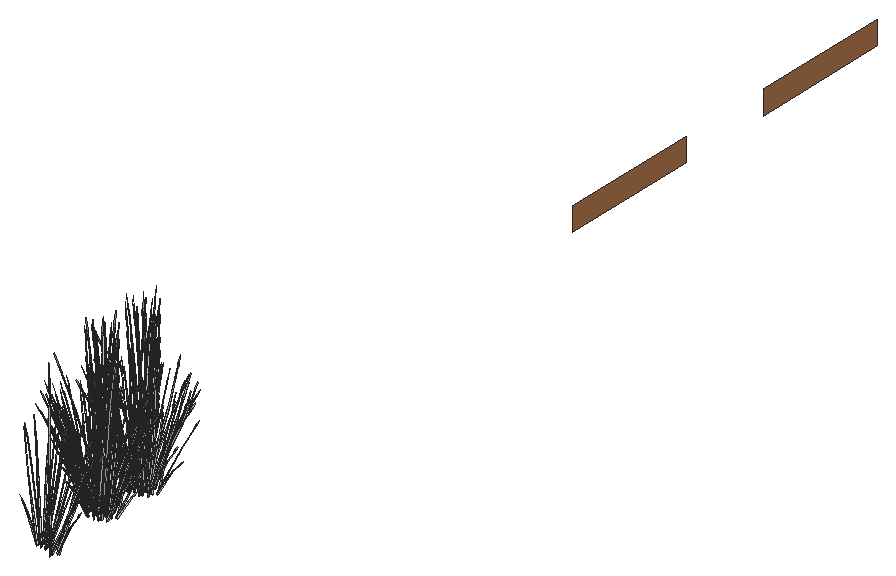
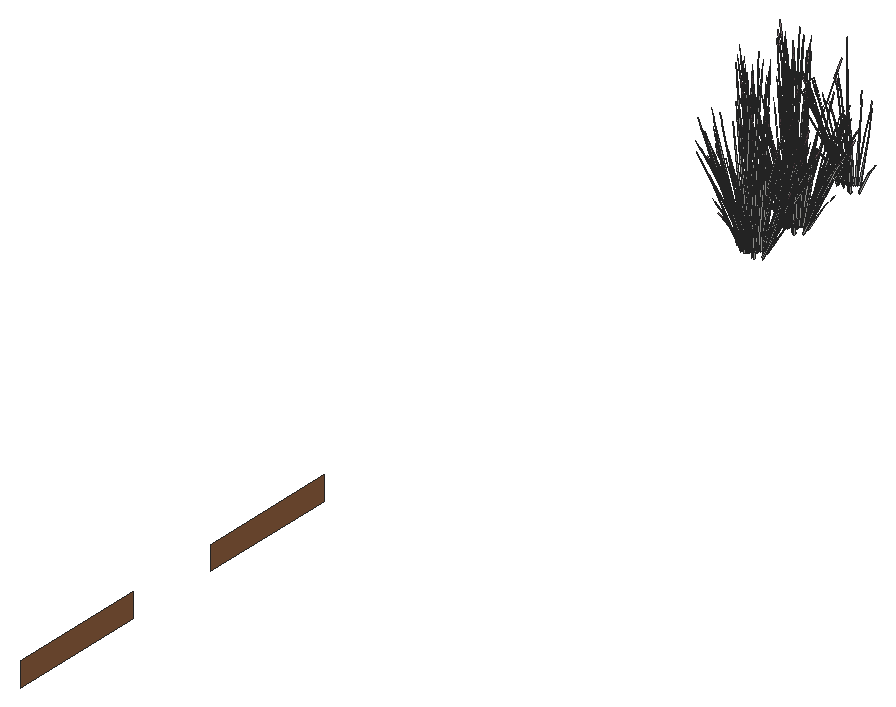
# SketchUp Ruby script. Lengths in inches.
U = 1.inch
M = Sketchup.active_model
def pt(a) = Geom::Point3d.new(a.map { |v| v * U })
def face(e, loops, mat)
  f = e.add_face(loops[0].map { |a| pt(a) })
  loops[1..].each { |l| e.add_face(l.map { |a| pt(a) }).erase! }
  f.material = f.back_material = mat if mat
  f
end
# faces: each face lists its corners as indices into pts; further lists are holes
def faces(e, pts, list, mat = nil) = list.each { |f| face(e, (f[0].is_a?(Array) ? f : [f]).map { |l| l.map { |i| pts[i] } }, mat) }
# xy, xz, yz: faces in a plane at the given z, y or x. An outline is a flat list of corners, or four numbers for a rectangle; further outlines are holes
def ring(l) = l.size == 4 ? [[l[0], l[1]], [l[2], l[1]], [l[2], l[3]], [l[0], l[3]]] : l.each_slice(2).to_a
def flat(e, list, mat, &to3) = list.each { |f| face(e, (f[0].is_a?(Array) ? f : [f]).map { |l| ring(l).map { |u, v| to3.(u, v) } }, mat) }
def xy(e, z, list, mat = nil) = flat(e, list, mat) { |x, y| [x, y, z] }
def xz(e, y, list, mat = nil) = flat(e, list, mat) { |x, z| [x, y, z] }
def yz(e, x, list, mat = nil) = flat(e, list, mat) { |y, z| [x, y, z] }
def lines(e, pts, list) = list.each { |a, b| e.add_line(pt(pts[a]), pt(pts[b])) }
# prism: a flat outline (further loops are holes) pulled along v
def prism(e, loops, v, mat = nil)
  f = face(e, loops, mat); d = Geom::Vector3d.new(v.map { |x| x * U })
  f.pushpull(f.normal.samedirection?(d) ? d.length : -d.length)
end
def box(e, o, s, mat = nil) = prism(e, [[o, [o[0] + s[0], o[1], o[2]], [o[0] + s[0], o[1] + s[1], o[2]], [o[0], o[1] + s[1], o[2]]]], [0, 0, s[2]], mat)
def at(x, y, z, deg = 0) = Geom::Transformation.translation(pt([x, y, z])) * Geom::Transformation.rotation(ORIGIN, Z_AXIS, deg.degrees)
def axes(o, x, y, z) = Geom::Transformation.new([*x, 0, *y, 0, *z, 0, *pt(o).to_a, 1])
def part(name) = M.definitions.add(name)
# library, detail: a bought-in or finely detailed component or shape, given as its bounding box
def library(name, o, s) = part(name).tap { |d| box(d.entities, o, s) }
def detail(e, o, s) = box(e.add_group.entities, o, s)
def put(e, d, t, mat = nil) = e.add_instance(d, t).tap { |i| i.material = mat if mat }
def group(e, t, mat = nil) = e.add_group.tap { |g| g.transformation = t; g.material = mat if mat }.entities
root = M.entities
M.materials.add("LightPink_Translucent").color = [144, 107, 117]
M.materials["LightPink_Translucent"].alpha = 0.75
M.materials.add("Wood_Veneer_15_1K").color = [163, 109, 71]
c1 = part("blade")
p = [[2.15,0.21,22],[0,0.17,0],[0.09,0.45,0],[2.18,0.31,22],[2.29,0.31,22],[0.38,0.45,0],
  [2.48,0.24,33],[2.49,0.24,33],[2.48,0.22,33]]
faces(c1.entities,p,[[0,1,2,3],[4,5,2,3],[6,3,4,7],[8,0,3,6]])
c2 = part("seeds")
p = [[0.3,-0.1,1.38],[-0.01,-0.03,1.59],[-0.01,-0.03,0.03],[0.14,-0.07,-0.07],[0.29,-0.03,3],[0.15,0.01,3.11]]
faces(c2.entities,p,[[0,1,2,3],[1,0,4,5]],"LightPink_Translucent")
c3 = part("blade with seeds")
put(c3.entities,c1,at(0,0,0))
put(c3.entities,c2,axes([2.4,0.25,30.99],[1.5799,-0.05474,1.17369],[-0.12525,1.92788,0.29478],[-0.07173,-0.02425,1.56792]))
yz(root,408,[[414.98,258.82,462.98,266.85],[495.98,258.82,543.98,266.85]],"Wood_Veneer_15_1K")
put(root,c3,axes([402.24,194.57,257.77],[0.31665,-0.27694,1.1486],[0.12495,0.43841,0.84392],[-0.22883,0.0785,0.25299]))
put(root,c3,axes([409.86,194.06,259.53],[0.43232,0.38257,-0.35414],[-0.49364,0.36215,0.4572],[0.25081,0.0551,0.87481]))
put(root,c3,axes([403.43,193.375,259.53],[-0.66138,0.08733,-0.35414],[-0.17464,-0.49921,0.4572],[-0.18953,0.13408,0.87481]))
put(root,c3,axes([408.31,193.08,258.875],[-0.28223,-0.10528,1.71376],[0.58406,-0.44165,0.13857],[0.36402,0.19924,0.73262]))
put(root,c3,axes([409.35,194.28,257.77],[-0.4278,-0.1757,1.1486],[0.5524,-0.17852,0.84392],[0.14899,0.15122,0.25299]))
put(root,c3,axes([404.58,192.88,258.875],[0.18977,-0.18775,1.71376],[0.47917,0.50677,0.13857],[-0.32866,0.23079,0.73262]))
put(root,c3,axes([403.98,193.43,259.68],[0.19519,0.55794,-0.51099],[-0.73919,0.0976,-0.3958],[-0.21183,0.14986,0.97773]))
put(root,c3,axes([408.3125,192.3,257.84],[-0.02076,-0.57531,1.41272],[0.93937,0.14913,0.59816],[-0.22217,0.31481,1.3335]))
put(root,c3,axes([408.39,194.52,259.68],[0.74975,-0.14525,-0.51099],[0.13115,0.55007,-0.3958],[0.20138,0.15763,0.97773]))
put(root,c3,axes([409.42,195.08,257.67],[-0.48723,-0.01916,1.0506],[0.32177,-0.40701,0.58006],[0.19248,0.1446,0.8241]))
put(root,c3,axes([404.43,193.35,258.875],[0.14147,-0.21002,1.71376],[0.59349,0.43464,0.13857],[-0.26773,0.27089,0.73262]))
put(root,c3,axes([407.83,194.09,257.59],[0.01341,-0.20255,1.43002],[0.64074,-0.22625,-0.30754],[0.1978,0.24243,0.61141]))
put(root,c3,axes([404.6,194.53,259.53],[-0.5141,0.32171,-0.35414],[-0.48666,-0.36734,0.4572],[-0.07405,0.18664,0.87481]))
put(root,c3,axes([404.92,195.78,257.77],[-0.01966,-0.36332,1.1486],[0.49135,0.25914,0.84392],[-0.09663,0.17317,0.25299]))
put(root,c3,axes([405.11,194.38,260],[0.54391,0.41056,-0.5672],[-0.57458,0.35956,-0.43934],[-0.08276,0.2086,1.08528]))
put(root,c3,axes([404.52,194.99,257.82],[0.69024,-0.1082,0.06507],[0.15868,0.43593,-0.86304],[-0.04376,0.22067,0.7736]))
put(root,c3,axes([406.72,194.78,259.68],[0.7469,0.15318,-0.51099],[-0.25601,0.52518,-0.3958],[0.06849,0.21144,0.97773]))
put(root,c3,axes([407.15,193.69,258.875],[-0.17368,-0.19618,1.71376],[0.80256,-0.16516,0.13857],[0.18139,0.30799,0.73262]))
put(root,c3,axes([406.38,195.1,259.53],[-0.22906,0.4699,-0.35414],[-0.66828,-0.13705,0.4572],[0.06128,0.18919,0.87481]))
put(root,c3,axes([404.94,194.19,260.34],[-0.01977,0.56521,-0.7886],[-0.83252,-0.03796,0.09517],[-0.08786,0.23945,1.11556]))
put(root,c3,axes([405.73,193.79,258.875],[-0.0186,-0.23452,1.71376],[0.80601,0.15558,0.13857],[-0.04985,0.33422,0.73262]))
put(root,c3,axes([406.45,194.68,259.98],[0.36264,0.49684,-0.71045],[-0.74649,0.27689,0.08574],[0.0848,0.24006,1.00501]))
put(root,c3,axes([404.35,195.46,257.59],[0.23977,-0.09639,1.43002],[0.59198,0.29065,-0.30754],[-0.1762,0.25149,0.61141]))
put(root,c3,axes([404.66,194.99,258.36],[0.01669,-0.31544,1.54345],[0.75083,0.16661,0.21329],[-0.06506,0.33618,0.72882]))
put(root,c3,axes([402.84,216.6,258.875],[0.17368,0.19618,1.71376],[-0.80256,0.16516,0.13857],[-0.18139,-0.30799,0.73262]))
put(root,c3,axes([405.96,216.32,257.59],[-0.21597,0.12368,1.43002],[-0.64681,-0.21647,-0.30754],[0.1199,-0.26922,0.61141]))
put(root,c3,axes([404.97,216.75,259.98],[-0.36264,-0.49684,-0.71045],[0.74649,-0.27689,0.08574],[-0.0848,-0.24006,1.00501]))
put(root,c3,axes([402.62,216.09,257.59],[-0.04601,0.19989,1.43002],[-0.67263,0.16733,-0.30754],[-0.15723,-0.25836,0.61141]))
put(root,c3,axes([406.48,217.24,259.98],[0.01977,-0.56521,-0.71045],[0.83252,0.03796,0.08574],[0.08786,-0.23945,1.00501]))
put(root,c3,axes([405.04,216.33,259.53],[0.22906,-0.4699,-0.35414],[0.66828,0.13705,0.4572],[-0.06128,-0.18919,0.87481]))
put(root,c3,axes([405.55,216.95,258.875],[-0.14147,0.21002,1.71376],[-0.59349,-0.43464,0.13857],[0.26773,-0.27089,0.73262]))
put(root,c3,axes([404.7,216.65,259.68],[-0.7469,-0.15318,-0.51099],[0.25601,-0.52518,-0.3958],[-0.06849,-0.21144,0.97773]))
put(root,c3,axes([405.16,215.34,257.77],[0.09747,0.35631,1.1486],[-0.54071,-0.19735,0.84392],[0.05818,-0.18244,0.25299]))
put(root,c3,axes([406.32,217.05,259.68],[-0.54391,-0.41056,-0.51099],[0.57458,-0.35956,-0.3958],[0.08276,-0.2086,0.97773]))
put(root,c3,axes([406.83,216.9,259.53],[0.5141,-0.32171,-0.35414],[0.48666,0.36734,0.4572],[0.07405,-0.18664,0.87481]))
put(root,c3,axes([402.38,215.76,257.77],[0.39634,0.21267,1.1486],[-0.57721,0.12784,0.84392],[-0.1235,-0.16344,0.25299]))
put(root,c3,axes([403.34,216.89,259.98],[-0.64788,-0.29534,-0.71045],[0.46044,-0.51755,0.08574],[-0.23473,-0.17635,1.00501]))
put(root,c3,axes([403.12,216.5,259.53],[-0.11735,-0.49217,-0.35414],[0.67083,-0.12996,0.4572],[-0.18018,-0.14104,0.87481]))
put(root,c3,axes([401.67,217.22,258.875],[0.28223,0.10528,1.71376],[-0.58406,0.44165,0.13857],[-0.36402,-0.19924,0.73262]))
put(root,c3,axes([403.04,216.91,259.68],[-0.74975,0.14525,-0.51099],[-0.13115,-0.55007,-0.3958],[-0.20138,-0.15763,0.97773]))
put(root,c3,axes([407.47,218.22,259.98],[0.39688,-0.48213,-0.71045],[0.69548,0.34264,0.08574],[0.23697,-0.17468,1.00501]))
put(root,c3,axes([407.45,217.99,259.68],[-0.19519,-0.55794,-0.51099],[0.73919,-0.0976,-0.3958],[0.21183,-0.14986,0.97773]))
put(root,c3,axes([404.89,220.23,258.33],[0.65659,0.2464,1.51261],[-0.64324,0.53082,0.59816],[-0.28812,-0.31461,1.26806]))
put(root,c3,axes([408.04,217.78,257.59],[-0.27143,-0.0181,1.43002],[-0.27808,-0.48551,-0.30754],[0.33346,-0.13735,0.61141]))
put(root,c3,axes([408.35,216.88,257.77],[-0.25308,0.31105,1.1486],[-0.21753,-0.4179,0.84392],[0.20902,-0.10472,0.25299]))
put(root,c3,axes([407.99,218.05,259.53],[0.66138,-0.08733,-0.35414],[0.17464,0.49921,0.4572],[0.18953,-0.13408,0.87481]))
put(root,c3,axes([401.5625,217.37,259.53],[-0.43232,-0.38257,-0.35414],[0.49364,-0.36215,0.4572],[-0.25081,-0.0551,0.87481]))
put(root,c3,axes([401.41,217.77,257.59],[0.14835,0.17012,1.43002],[-0.34183,0.46242,-0.30754],[-0.351,-0.11053,0.61141]))
put(root,c3,axes([402.02,217.62,259.98],[-0.75952,-0.01471,-0.71045],[0.05101,-0.61953,0.08574],[-0.32177,-0.06538,1.00501]))
put(root,c3,axes([404.23,219.05,257.43],[0.8561,0.29616,0.24065],[-0.41201,0.61537,0.50002],[0,-0.14185,1.60543]))
put(root,c3,axes([401.77,217.75,259.68],[-0.55171,0.40476,-0.51099],[-0.48318,-0.42758,-0.3958],[-0.28031,-0.06159,0.97773]))
put(root,c3,axes([400.52,218.28,257.77],[0.48508,-0.04372,1.1486],[-0.3077,0.38525,0.84392],[-0.23971,-0.05779,0.25299]))
put(root,c3,axes([403.95,218.64,257.72],[-0.82508,0.03772,0.44739],[-0.07462,-0.62614,-0.21531],[0.14771,-0.06346,1.43643]))
put(root,c3,axes([401.82,219.1,257.48],[0,0.61104,0.49651],[-0.85008,0,0],[0,-0.13917,1.57504]))
put(root,c3,axes([407.79,219.23,259.68],[0.20584,-0.55581,-0.51099],[0.70573,0.19051,-0.3958],[0.28414,-0.05097,0.97773]))
put(root,c3,axes([401.08,218.18,258.875],[0.31515,-0.01384,1.71376],[-0.20907,0.5998,0.13857],[-0.44912,-0.0371,0.73262]))
put(root,c3,axes([403.76,219.4,257.72],[-0.36864,0.55059,0.44739],[-0.76598,-0.26498,-0.21531],[0,-0.12692,1.43643]))
put(root,c3,axes([406.26,217.29,257.48],[-0.7111,-0.30552,0.49651],[0.42504,-0.54784,0],[0.16196,0.06958,1.57504]))
put(root,c3,axes([407.65,219.44,259.98],[0.66765,-0.26986,-0.71045],[0.37208,0.55551,0.08574],[0.32259,-0.0631,1.00501]))
put(root,c3,axes([403.57,217.56,257.47],[-0.21949,0.60727,0.17642],[-0.8032,-0.17185,0.35086],[0.13875,-0.00296,1.60407]))
put(root,c3,axes([405.25,218.24,257.62],[0.14658,-0.54532,0.1448],[0.71613,0.09466,-0.41347],[0.13033,0.05599,1.26744]))
put(root,c3,axes([404.9375,218.38,257.72],[-0.45644,-0.51287,0.44739],[0.69137,-0.36116,-0.21531],[0.14771,0.06346,1.43643]))
put(root,c3,axes([403.49,220.7,257.47],[0.81646,-0.16218,0.17642],[0.20161,0.60355,0.35086],[-0.07282,-0.08794,1.60407]))
put(root,c3,axes([408.22,219.49,259.53],[0.63144,0.17046,-0.35414],[-0.18417,0.49731,0.4572],[0.25423,-0.0456,0.87481]))
put(root,c3,axes([400.8,218.69,259.53],[-0.63144,-0.17046,-0.35414],[0.18417,-0.49731,0.4572],[-0.25423,0.0456,0.87481]))
put(root,c3,axes([406,217.6,257.47],[-0.81646,0.16218,0.17642],[-0.20161,-0.60355,0.35086],[0.07282,0.08794,1.60407]))
put(root,c3,axes([406.5,218.87,258.875],[-0.31515,0.01384,1.71376],[0.20907,-0.5998,0.13857],[0.44912,0.0371,0.73262]))
put(root,c3,axes([405.48,218.76,257.38],[-0.96033,-0.12874,0.49198],[0.19544,-0.7271,0.19306],[0.14034,0.07021,1.70813]))
put(root,c3,axes([404.24,220.05,257.62],[-0.14658,0.54532,0.1448],[-0.71613,-0.09466,-0.41347],[-0.13033,-0.05599,1.26744]))
put(root,c3,axes([405.92,220.73,257.47],[0.21949,-0.60727,0.17642],[0.8032,0.17185,0.35086],[-0.13875,0.00296,1.60407]))
put(root,c3,axes([402.72,218.61,258.34],[0.21597,-0.08839,1.77064],[0.07448,0.61717,0.13857],[-0.4678,0.08189,0.63284]))
put(root,c3,axes([407.17,219.18,257.47],[-0.59697,-0.44509,0.17642],[0.60159,-0.4317,0.35086],[-0.06593,0.0909,1.60407]))
put(root,c3,axes([409.5625,219.59,257.77],[-0.46945,0.10088,1.1486],[0.22097,-0.4169,0.84392],[0.24904,0.02853,0.25299]))
put(root,c3,axes([403.22,221,257.48],[0.7111,0.30552,0.49651],[-0.42504,0.54784,0],[-0.16196,-0.06958,1.57504]))
put(root,c3,axes([405.73,218.89,257.72],[0.36864,-0.55059,0.44739],[0.76598,0.26498,-0.21531],[0,0.12692,1.43643]))
put(root,c3,axes([401.23,218.95,259.68],[-0.20584,0.55581,-0.51099],[-0.70573,-0.19051,-0.3958],[-0.28414,0.05097,0.97773]))
put(root,c3,axes([408.75,220.87,258.93],[-0.14542,-0.51365,-0.03492],[0.68734,-0.11809,-0.15832],[0.14353,0.03256,0.52218]))
put(root,c3,axes([407.67,219.2,257.48],[0,-0.61104,0.49651],[0.85008,0,0],[0,0.13917,1.57504]))
put(root,c3,axes([405.54,219.65,257.72],[0.82508,-0.03772,0.44739],[0.07462,0.62614,-0.21531],[-0.14771,0.06346,1.43643]))
put(root,c3,axes([406.05,219.02,257.62],[0.70791,-0.1782,0.1448],[0.24791,0.50885,-0.41347],[0,0.11199,1.26744]))
put(root,c3,axes([408.68,220.26,257.59],[-0.18299,-0.15028,1.43002],[0.23809,-0.49714,-0.30754],[0.37023,0.06735,0.61141]))
put(root,c3,axes([405.55,219.92,257.62],[0.56134,0.36712,0.1448],[-0.46823,0.41419,-0.41347],[-0.13033,0.05599,1.26744]))
put(root,c3,axes([401.21,219.23,258.875],[0.26363,-0.12925,1.71376],[0.22195,0.59723,0.13857],[-0.41388,0.13498,0.73262]))
put(root,c3,axes([407,220.56,259.98],[0.75952,0.01471,-0.71045],[-0.05101,0.61953,0.08574],[0.32177,0.06538,1.00501]))
put(root,c3,axes([406.15,221.06,257.48],[0.7111,-0.30552,0.49651],[0.42504,0.54784,0],[-0.16196,0.06958,1.57504]))
put(root,c3,axes([400.39,220.25,257.59],[0.26405,0.05016,1.43002],[0.17019,0.51235,-0.30754],[-0.35868,0.0959,0.61141]))
put(root,c3,axes([399.84,221.33,257.77],[0.31665,-0.27694,1.1486],[0.12495,0.43841,0.84392],[-0.22883,0.0785,0.25299]))
put(root,c3,axes([407.46,220.8125,259.53],[0.43232,0.38257,-0.35414],[-0.49364,0.36215,0.4572],[0.25081,0.0551,0.87481]))
put(root,c3,axes([401.03,220.13,259.53],[-0.66138,0.08733,-0.35414],[-0.17464,-0.49921,0.4572],[-0.18953,0.13408,0.87481]))
put(root,c3,axes([405.91,219.83,258.875],[-0.28223,-0.10528,1.71376],[0.58406,-0.44165,0.13857],[0.36402,0.19924,0.73262]))
put(root,c3,axes([406.95,221.03,257.77],[-0.4278,-0.1757,1.1486],[0.5524,-0.17852,0.84392],[0.14899,0.15122,0.25299]))
put(root,c3,axes([402.17,219.64,258.875],[0.18977,-0.18775,1.71376],[0.47917,0.50677,0.13857],[-0.32866,0.23079,0.73262]))
put(root,c3,axes([401.58,220.1875,259.68],[0.19519,0.55794,-0.51099],[-0.73919,0.0976,-0.3958],[-0.21183,0.14986,0.97773]))
put(root,c3,axes([405.91,219.06,257.84],[-0.02076,-0.57531,1.41272],[0.93937,0.14913,0.59816],[-0.22217,0.31481,1.3335]))
put(root,c3,axes([405.98,221.27,259.68],[0.74975,-0.14525,-0.51099],[0.13115,0.55007,-0.3958],[0.20138,0.15763,0.97773]))
put(root,c3,axes([407.02,221.83,257.67],[-0.48723,-0.01916,1.0506],[0.32177,-0.40701,0.58006],[0.19248,0.1446,0.8241]))
put(root,c3,axes([402.03,220.1,258.875],[0.14147,-0.21002,1.71376],[0.59349,0.43464,0.13857],[-0.26773,0.27089,0.73262]))
put(root,c3,axes([405.43,220.85,257.59],[0.01341,-0.20255,1.43002],[0.64074,-0.22625,-0.30754],[0.1978,0.24243,0.61141]))
put(root,c3,axes([402.19,221.28,259.53],[-0.5141,0.32171,-0.35414],[-0.48666,-0.36734,0.4572],[-0.07405,0.18664,0.87481]))
put(root,c3,axes([402.52,222.53,257.77],[-0.01966,-0.36332,1.1486],[0.49135,0.25914,0.84392],[-0.09663,0.17317,0.25299]))
put(root,c3,axes([402.71,221.13,260],[0.54391,0.41056,-0.5672],[-0.57458,0.35956,-0.43934],[-0.08276,0.2086,1.08528]))
put(root,c3,axes([402.12,221.75,257.82],[0.69024,-0.1082,0.06507],[0.15868,0.43593,-0.86304],[-0.04376,0.22067,0.7736]))
put(root,c3,axes([404.32,221.53,259.68],[0.7469,0.15318,-0.51099],[-0.25601,0.52518,-0.3958],[0.06849,0.21144,0.97773]))
put(root,c3,axes([404.74,220.45,258.875],[-0.17368,-0.19618,1.71376],[0.80256,-0.16516,0.13857],[0.18139,0.30799,0.73262]))
put(root,c3,axes([403.98,221.85,259.53],[-0.22906,0.4699,-0.35414],[-0.66828,-0.13705,0.4572],[0.06128,0.18919,0.87481]))
put(root,c3,axes([402.54,220.94,260.34],[-0.01977,0.56521,-0.7886],[-0.83252,-0.03796,0.09517],[-0.08786,0.23945,1.11556]))
put(root,c3,axes([403.32,220.54,258.875],[-0.0186,-0.23452,1.71376],[0.80601,0.15558,0.13857],[-0.04985,0.33422,0.73262]))
put(root,c3,axes([404.05,221.43,259.98],[0.36264,0.49684,-0.71045],[-0.74649,0.27689,0.08574],[0.0848,0.24006,1.00501]))
put(root,c3,axes([401.95,222.21,257.59],[0.23977,-0.09639,1.43002],[0.59198,0.29065,-0.30754],[-0.1762,0.25149,0.61141]))
put(root,c3,axes([402.26,221.74,258.36],[0.01669,-0.31544,1.54345],[0.75083,0.16661,0.21329],[-0.06506,0.33618,0.72882]))
put(root,c3,axes([402.99,233.67,258.875],[0.17368,0.19618,1.71376],[-0.80256,0.16516,0.13857],[-0.18139,-0.30799,0.73262]))
put(root,c3,axes([406.12,233.39,257.59],[-0.21597,0.12368,1.43002],[-0.64681,-0.21647,-0.30754],[0.1199,-0.26922,0.61141]))
put(root,c3,axes([405.13,233.82,259.98],[-0.36264,-0.49684,-0.71045],[0.74649,-0.27689,0.08574],[-0.0848,-0.24006,1.00501]))
put(root,c3,axes([402.77,233.16,257.59],[-0.04601,0.19989,1.43002],[-0.67263,0.16733,-0.30754],[-0.15723,-0.25836,0.61141]))
put(root,c3,axes([406.64,234.31,259.98],[0.01977,-0.56521,-0.71045],[0.83252,0.03796,0.08574],[0.08786,-0.23945,1.00501]))
put(root,c3,axes([405.2,233.4,259.53],[0.22906,-0.4699,-0.35414],[0.66828,0.13705,0.4572],[-0.06128,-0.18919,0.87481]))
put(root,c3,axes([405.71,234.02,258.875],[-0.14147,0.21002,1.71376],[-0.59349,-0.43464,0.13857],[0.26773,-0.27089,0.73262]))
put(root,c3,axes([404.86,233.72,259.68],[-0.7469,-0.15318,-0.51099],[0.25601,-0.52518,-0.3958],[-0.06849,-0.21144,0.97773]))
put(root,c3,axes([405.32,232.41,257.77],[0.09747,0.35631,1.1486],[-0.54071,-0.19735,0.84392],[0.05818,-0.18244,0.25299]))
put(root,c3,axes([406.47,234.12,259.68],[-0.54391,-0.41056,-0.51099],[0.57458,-0.35956,-0.3958],[0.08276,-0.2086,0.97773]))
put(root,c3,axes([406.99,233.97,259.53],[0.5141,-0.32171,-0.35414],[0.48666,0.36734,0.4572],[0.07405,-0.18664,0.87481]))
put(root,c3,axes([402.54,232.83,257.77],[0.39634,0.21267,1.1486],[-0.57721,0.12784,0.84392],[-0.1235,-0.16344,0.25299]))
put(root,c3,axes([403.5,233.96,259.98],[-0.64788,-0.29534,-0.71045],[0.46044,-0.51755,0.08574],[-0.23473,-0.17635,1.00501]))
put(root,c3,axes([403.27,233.57,259.53],[-0.11735,-0.49217,-0.35414],[0.67083,-0.12996,0.4572],[-0.18018,-0.14104,0.87481]))
put(root,c3,axes([401.83,234.29,258.875],[0.28223,0.10528,1.71376],[-0.58406,0.44165,0.13857],[-0.36402,-0.19924,0.73262]))
put(root,c3,axes([403.2,233.98,259.68],[-0.74975,0.14525,-0.51099],[-0.13115,-0.55007,-0.3958],[-0.20138,-0.15763,0.97773]))
put(root,c3,axes([407.625,235.29,259.98],[0.39688,-0.48213,-0.71045],[0.69548,0.34264,0.08574],[0.23697,-0.17468,1.00501]))
put(root,c3,axes([407.6,235.06,259.68],[-0.19519,-0.55794,-0.51099],[0.73919,-0.0976,-0.3958],[0.21183,-0.14986,0.97773]))
put(root,c3,axes([405.05,237.3,258.33],[0.65659,0.2464,1.51261],[-0.64324,0.53082,0.59816],[-0.28812,-0.31461,1.26806]))
put(root,c3,axes([408.2,234.85,257.59],[-0.27143,-0.0181,1.43002],[-0.27808,-0.48551,-0.30754],[0.33346,-0.13735,0.61141]))
put(root,c3,axes([408.51,233.95,257.77],[-0.25308,0.31105,1.1486],[-0.21753,-0.4179,0.84392],[0.20902,-0.10472,0.25299]))
put(root,c3,axes([408.15,235.125,259.53],[0.66138,-0.08733,-0.35414],[0.17464,0.49921,0.4572],[0.18953,-0.13408,0.87481]))
put(root,c3,axes([401.72,234.4375,259.53],[-0.43232,-0.38257,-0.35414],[0.49364,-0.36215,0.4572],[-0.25081,-0.0551,0.87481]))
put(root,c3,axes([401.57,234.84,257.59],[0.14835,0.17012,1.43002],[-0.34183,0.46242,-0.30754],[-0.351,-0.11053,0.61141]))
put(root,c3,axes([402.18,234.69,259.98],[-0.75952,-0.01471,-0.71045],[0.05101,-0.61953,0.08574],[-0.32177,-0.06538,1.00501]))
put(root,c3,axes([404.39,236.12,257.43],[0.8561,0.29616,0.24065],[-0.41201,0.61537,0.50002],[0,-0.14185,1.60543]))
put(root,c3,axes([401.93,234.82,259.68],[-0.55171,0.40476,-0.51099],[-0.48318,-0.42758,-0.3958],[-0.28031,-0.06159,0.97773]))
put(root,c3,axes([400.68,235.35,257.77],[0.48508,-0.04372,1.1486],[-0.3077,0.38525,0.84392],[-0.23971,-0.05779,0.25299]))
put(root,c3,axes([404.11,235.71,257.72],[-0.82508,0.03772,0.44739],[-0.07462,-0.62614,-0.21531],[0.14771,-0.06346,1.43643]))
put(root,c3,axes([401.98,236.17,257.48],[0,0.61104,0.49651],[-0.85008,0,0],[0,-0.13917,1.57504]))
put(root,c3,axes([407.95,236.3,259.68],[0.20584,-0.55581,-0.51099],[0.70573,0.19051,-0.3958],[0.28414,-0.05097,0.97773]))
put(root,c3,axes([401.24,235.25,258.875],[0.31515,-0.01384,1.71376],[-0.20907,0.5998,0.13857],[-0.44912,-0.0371,0.73262]))
put(root,c3,axes([403.92,236.47,257.72],[-0.36864,0.55059,0.44739],[-0.76598,-0.26498,-0.21531],[0,-0.12692,1.43643]))
put(root,c3,axes([406.42,234.36,257.48],[-0.7111,-0.30552,0.49651],[0.42504,-0.54784,0],[0.16196,0.06958,1.57504]))
put(root,c3,axes([407.8125,236.51,259.98],[0.66765,-0.26986,-0.71045],[0.37208,0.55551,0.08574],[0.32259,-0.0631,1.00501]))
put(root,c3,axes([403.73,234.64,257.47],[-0.21949,0.60727,0.17642],[-0.8032,-0.17185,0.35086],[0.13875,-0.00296,1.60407]))
put(root,c3,axes([405.4,235.31,257.62],[0.14658,-0.54532,0.1448],[0.71613,0.09466,-0.41347],[0.13033,0.05599,1.26744]))
put(root,c3,axes([405.1,235.45,257.72],[-0.45644,-0.51287,0.44739],[0.69137,-0.36116,-0.21531],[0.14771,0.06346,1.43643]))
put(root,c3,axes([403.65,237.77,257.47],[0.81646,-0.16218,0.17642],[0.20161,0.60355,0.35086],[-0.07282,-0.08794,1.60407]))
put(root,c3,axes([408.38,236.56,259.53],[0.63144,0.17046,-0.35414],[-0.18417,0.49731,0.4572],[0.25423,-0.0456,0.87481]))
put(root,c3,axes([400.96,235.76,259.53],[-0.63144,-0.17046,-0.35414],[0.18417,-0.49731,0.4572],[-0.25423,0.0456,0.87481]))
put(root,c3,axes([406.16,234.67,257.47],[-0.81646,0.16218,0.17642],[-0.20161,-0.60355,0.35086],[0.07282,0.08794,1.60407]))
put(root,c3,axes([406.66,235.94,258.875],[-0.31515,0.01384,1.71376],[0.20907,-0.5998,0.13857],[0.44912,0.0371,0.73262]))
put(root,c3,axes([405.64,235.83,257.38],[-0.96033,-0.12874,0.49198],[0.19544,-0.7271,0.19306],[0.14034,0.07021,1.70813]))
put(root,c3,axes([404.4,237.125,257.62],[-0.14658,0.54532,0.1448],[-0.71613,-0.09466,-0.41347],[-0.13033,-0.05599,1.26744]))
put(root,c3,axes([406.08,237.8,257.47],[0.21949,-0.60727,0.17642],[0.8032,0.17185,0.35086],[-0.13875,0.00296,1.60407]))
put(root,c3,axes([402.88,235.68,258.34],[0.21597,-0.08839,1.77064],[0.07448,0.61717,0.13857],[-0.4678,0.08189,0.63284]))
put(root,c3,axes([407.33,236.25,257.47],[-0.59697,-0.44509,0.17642],[0.60159,-0.4317,0.35086],[-0.06593,0.0909,1.60407]))
put(root,c3,axes([409.72,236.66,257.77],[-0.46945,0.10088,1.1486],[0.22097,-0.4169,0.84392],[0.24904,0.02853,0.25299]))
put(root,c3,axes([403.38,238.08,257.48],[0.7111,0.30552,0.49651],[-0.42504,0.54784,0],[-0.16196,-0.06958,1.57504]))
put(root,c3,axes([405.89,235.96,257.72],[0.36864,-0.55059,0.44739],[0.76598,0.26498,-0.21531],[0,0.12692,1.43643]))
put(root,c3,axes([401.39,236.02,259.68],[-0.20584,0.55581,-0.51099],[-0.70573,-0.19051,-0.3958],[-0.28414,0.05097,0.97773]))
put(root,c3,axes([408.9,237.94,258.93],[-0.14542,-0.51365,-0.03492],[0.68734,-0.11809,-0.15832],[0.14353,0.03256,0.52218]))
put(root,c3,axes([407.82,236.27,257.48],[0,-0.61104,0.49651],[0.85008,0,0],[0,0.13917,1.57504]))
put(root,c3,axes([405.69,236.73,257.72],[0.82508,-0.03772,0.44739],[0.07462,0.62614,-0.21531],[-0.14771,0.06346,1.43643]))
put(root,c3,axes([406.21,236.09,257.62],[0.70791,-0.1782,0.1448],[0.24791,0.50885,-0.41347],[0,0.11199,1.26744]))
put(root,c3,axes([408.84,237.33,257.59],[-0.18299,-0.15028,1.43002],[0.23809,-0.49714,-0.30754],[0.37023,0.06735,0.61141]))
put(root,c3,axes([405.71,236.99,257.62],[0.56134,0.36712,0.1448],[-0.46823,0.41419,-0.41347],[-0.13033,0.05599,1.26744]))
put(root,c3,axes([401.37,236.31,258.875],[0.26363,-0.12925,1.71376],[0.22195,0.59723,0.13857],[-0.41388,0.13498,0.73262]))
put(root,c3,axes([407.16,237.63,259.98],[0.75952,0.01471,-0.71045],[-0.05101,0.61953,0.08574],[0.32177,0.06538,1.00501]))
put(root,c3,axes([406.3,238.125,257.48],[0.7111,-0.30552,0.49651],[0.42504,0.54784,0],[-0.16196,0.06958,1.57504]))
put(root,c3,axes([400.55,237.32,257.59],[0.26405,0.05016,1.43002],[0.17019,0.51235,-0.30754],[-0.35868,0.0959,0.61141]))
put(root,c3,axes([400,238.4,257.77],[0.31665,-0.27694,1.1486],[0.12495,0.43841,0.84392],[-0.22883,0.0785,0.25299]))
put(root,c3,axes([407.62,237.88,259.53],[0.43232,0.38257,-0.35414],[-0.49364,0.36215,0.4572],[0.25081,0.0551,0.87481]))
put(root,c3,axes([401.1875,237.2,259.53],[-0.66138,0.08733,-0.35414],[-0.17464,-0.49921,0.4572],[-0.18953,0.13408,0.87481]))
put(root,c3,axes([406.0625,236.9,258.875],[-0.28223,-0.10528,1.71376],[0.58406,-0.44165,0.13857],[0.36402,0.19924,0.73262]))
put(root,c3,axes([407.11,238.1,257.77],[-0.4278,-0.1757,1.1486],[0.5524,-0.17852,0.84392],[0.14899,0.15122,0.25299]))
put(root,c3,axes([402.33,236.71,258.875],[0.18977,-0.18775,1.71376],[0.47917,0.50677,0.13857],[-0.32866,0.23079,0.73262]))
put(root,c3,axes([401.73,237.26,259.68],[0.19519,0.55794,-0.51099],[-0.73919,0.0976,-0.3958],[-0.21183,0.14986,0.97773]))
put(root,c3,axes([406.07,236.125,257.84],[-0.02076,-0.57531,1.41272],[0.93937,0.14913,0.59816],[-0.22217,0.31481,1.3335]))
put(root,c3,axes([406.14,238.34,259.68],[0.74975,-0.14525,-0.51099],[0.13115,0.55007,-0.3958],[0.20138,0.15763,0.97773]))
put(root,c3,axes([407.18,238.9,257.67],[-0.48723,-0.01916,1.0506],[0.32177,-0.40701,0.58006],[0.19248,0.1446,0.8241]))
put(root,c3,axes([402.1875,237.17,258.875],[0.14147,-0.21002,1.71376],[0.59349,0.43464,0.13857],[-0.26773,0.27089,0.73262]))
put(root,c3,axes([405.59,237.92,257.59],[0.01341,-0.20255,1.43002],[0.64074,-0.22625,-0.30754],[0.1978,0.24243,0.61141]))
put(root,c3,axes([402.35,238.35,259.53],[-0.5141,0.32171,-0.35414],[-0.48666,-0.36734,0.4572],[-0.07405,0.18664,0.87481]))
put(root,c3,axes([402.68,239.6,257.77],[-0.01966,-0.36332,1.1486],[0.49135,0.25914,0.84392],[-0.09663,0.17317,0.25299]))
put(root,c3,axes([402.86,238.2,260],[0.54391,0.41056,-0.5672],[-0.57458,0.35956,-0.43934],[-0.08276,0.2086,1.08528]))
put(root,c3,axes([402.27,238.82,257.82],[0.69024,-0.1082,0.06507],[0.15868,0.43593,-0.86304],[-0.04376,0.22067,0.7736]))
put(root,c3,axes([404.48,238.6,259.68],[0.7469,0.15318,-0.51099],[-0.25601,0.52518,-0.3958],[0.06849,0.21144,0.97773]))
put(root,c3,axes([404.9,237.52,258.875],[-0.17368,-0.19618,1.71376],[0.80256,-0.16516,0.13857],[0.18139,0.30799,0.73262]))
put(root,c3,axes([404.14,238.92,259.53],[-0.22906,0.4699,-0.35414],[-0.66828,-0.13705,0.4572],[0.06128,0.18919,0.87481]))
put(root,c3,axes([402.7,238.01,260.34],[-0.01977,0.56521,-0.7886],[-0.83252,-0.03796,0.09517],[-0.08786,0.23945,1.11556]))
put(root,c3,axes([403.48,237.61,258.875],[-0.0186,-0.23452,1.71376],[0.80601,0.15558,0.13857],[-0.04985,0.33422,0.73262]))
put(root,c3,axes([404.21,238.5,259.98],[0.36264,0.49684,-0.71045],[-0.74649,0.27689,0.08574],[0.0848,0.24006,1.00501]))
put(root,c3,axes([402.11,239.28,257.59],[0.23977,-0.09639,1.43002],[0.59198,0.29065,-0.30754],[-0.1762,0.25149,0.61141]))
put(root,c3,axes([402.42,238.8125,258.36],[0.01669,-0.31544,1.54345],[0.75083,0.16661,0.21329],[-0.06506,0.33618,0.72882]))
